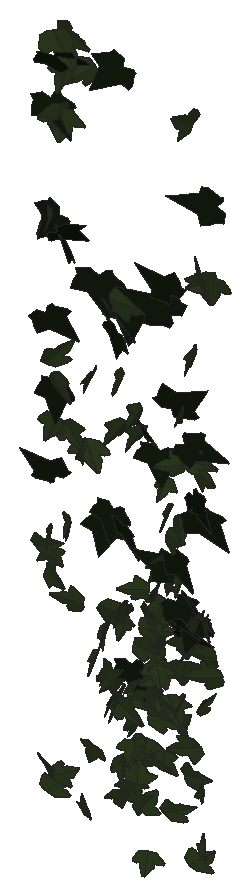
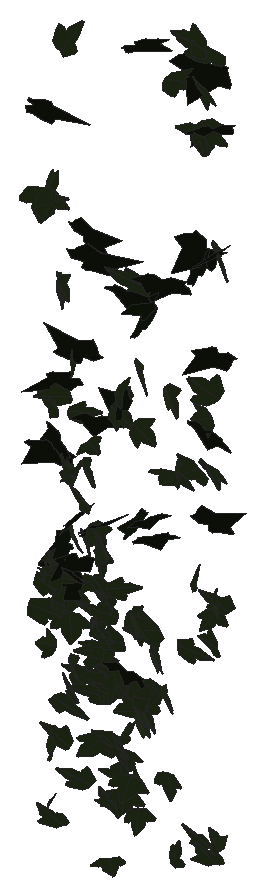
# SketchUp Ruby script. Lengths in inches.
U = 1.inch
M = Sketchup.active_model
def pt(a) = Geom::Point3d.new(a.map { |v| v * U })
def face(e, loops, mat)
  f = e.add_face(loops[0].map { |a| pt(a) })
  loops[1..].each { |l| e.add_face(l.map { |a| pt(a) }).erase! }
  f.material = f.back_material = mat if mat
  f
end
# faces: each face lists its corners as indices into pts; further lists are holes
def faces(e, pts, list, mat = nil) = list.each { |f| face(e, (f[0].is_a?(Array) ? f : [f]).map { |l| l.map { |i| pts[i] } }, mat) }
# xy, xz, yz: faces in a plane at the given z, y or x. An outline is a flat list of corners, or four numbers for a rectangle; further outlines are holes
def ring(l) = l.size == 4 ? [[l[0], l[1]], [l[2], l[1]], [l[2], l[3]], [l[0], l[3]]] : l.each_slice(2).to_a
def flat(e, list, mat, &to3) = list.each { |f| face(e, (f[0].is_a?(Array) ? f : [f]).map { |l| ring(l).map { |u, v| to3.(u, v) } }, mat) }
def xy(e, z, list, mat = nil) = flat(e, list, mat) { |x, y| [x, y, z] }
def xz(e, y, list, mat = nil) = flat(e, list, mat) { |x, z| [x, y, z] }
def yz(e, x, list, mat = nil) = flat(e, list, mat) { |y, z| [x, y, z] }
def lines(e, pts, list) = list.each { |a, b| e.add_line(pt(pts[a]), pt(pts[b])) }
# prism: a flat outline (further loops are holes) pulled along v
def prism(e, loops, v, mat = nil)
  f = face(e, loops, mat); d = Geom::Vector3d.new(v.map { |x| x * U })
  f.pushpull(f.normal.samedirection?(d) ? d.length : -d.length)
end
def box(e, o, s, mat = nil) = prism(e, [[o, [o[0] + s[0], o[1], o[2]], [o[0] + s[0], o[1] + s[1], o[2]], [o[0], o[1] + s[1], o[2]]]], [0, 0, s[2]], mat)
def at(x, y, z, deg = 0) = Geom::Transformation.translation(pt([x, y, z])) * Geom::Transformation.rotation(ORIGIN, Z_AXIS, deg.degrees)
def axes(o, x, y, z) = Geom::Transformation.new([*x, 0, *y, 0, *z, 0, *pt(o).to_a, 1])
def part(name) = M.definitions.add(name)
# library, detail: a bought-in or finely detailed component or shape, given as its bounding box
def library(name, o, s) = part(name).tap { |d| box(d.entities, o, s) }
def detail(e, o, s) = box(e.add_group.entities, o, s)
def put(e, d, t, mat = nil) = e.add_instance(d, t).tap { |i| i.material = mat if mat }
def group(e, t, mat = nil) = e.add_group.tap { |g| g.transformation = t; g.material = mat if mat }.entities
root = M.entities
M.materials.add("1026 AP 7946 SUNNY SIDE UP").color = [254, 231, 186]
M.materials.add("efeu1").color = [18, 25, 13]
M.materials.add("efeu2").color = [43, 57, 29]
c1 = part("ivyleaf_10")
p = [[0,0.5,-0.03],[-0.0625,2.02,-0.43],[-0.19,2.01,-0.46],[-0.54,1.05,-0.29],[-0.52,0.625,-0.18],[-0.83,0.76,-0.28],
  [-1.16,0.64,-0.33],[-1.15,0.33,-0.24],[-0.77,-0.39,0.02],[-0.3,-0.51,0.16],[0.04,-0.48,0.23],[-0.02,2.01,-0.4375],
  [-0.06,2.01,-0.43],[0.04,-0.49,0.23],[0.67,-0.49,0.14],[1.38,0.36,-0.2],[1.375,0.51,-0.24],[0.81,0.65,-0.19],
  [0.62,0.59,-0.15],[0.6,1.09,-0.28],[0.5,1.23,-0.31]]
faces(c1.entities,p,[[0,1,2,3,4,5,6,7,8,9,10],[11,12,0,13,14,15,16,17,18,19,20]],"efeu2")
c2 = part("ivyleaf_9")
p = [[1.54,2.16,1.25],[1.36,2.04,1.19],[-0.21,0.99,0.68],[-0.71,1.11,0.82],[-0.85,0.86,0.67],[-0.8,0.17,0.21],
  [-0.9,-0.01,0.1],[-0.67,-0.16,-0.02],[-0.08,-0.08,-0.05],[-0.03,-0.6,-0.4],[0.65,-0.88,-0.66],[0.83,-0.6,-0.49],
  [1.29,-0.42,-0.43],[1.8125,-0.07,-0.26],[1.21,0.44,0.15]]
faces(c2.entities,p,[[0,1,2,3,4,5,6,7,8,9,10,11,12,13,14]],"efeu1")
put(root,c1,axes([100.51,211.74,258.84],[-0.19659,0.09417,-0.18867],[0.19544,-0.13675,-0.16004],[-0.27947,-0.16188,0.0208]),"1026 AP 7946 SUNNY SIDE UP")
put(root,c1,axes([102.18,211.78,250.18],[0.2178,-0.07618,0.1738],[0.20785,-0.10757,-0.16206],[0.20465,0.19032,-0.02038]),"1026 AP 7946 SUNNY SIDE UP")
put(root,c1,axes([101.13,211.85,257.35],[-0.00488,-0.00097,-0.24211],[0.01134,-0.23492,-0.00047],[-0.36936,-0.0072,0.00319]),"1026 AP 7946 SUNNY SIDE UP")
put(root,c1,axes([104.76,211.65,253.64],[-0.07726,0.03119,0.21181],[-0.32666,-0.00394,-0.0506],[-0.00532,-0.21118,0.03096]),"1026 AP 7946 SUNNY SIDE UP")
put(root,c2,axes([103.46,211.8,255.27],[-0.09173,-0.23488,-0.0616],[-0.03309,-0.05498,0.24889],[-0.37914,0.06162,-0.00682]),"1026 AP 7946 SUNNY SIDE UP")
put(root,c1,axes([103.75,211.82,257.87],[-0.05406,0.02333,0.2117],[-0.12965,-0.19245,0.00718],[0.29801,-0.07949,0.04153]),"1026 AP 7946 SUNNY SIDE UP")
put(root,c1,axes([103.39,211.79,254.14],[0.1072,0.13302,-0.14483],[-0.08052,-0.13217,-0.15436],[-0.29437,0.08459,-0.01052]),"1026 AP 7946 SUNNY SIDE UP")
put(root,c1,axes([103.19,211.73,251.99],[-0.02244,0.00487,0.21035],[0.32049,-0.01245,0.01491],[0.02007,0.20428,-0.00291]),"1026 AP 7946 SUNNY SIDE UP")
put(root,c1,axes([104.73,211.79,253.09],[-0.07638,-0.01767,0.24407],[-0.28841,-0.15106,-0.05121],[0.23767,-0.18899,0.01629]),"1026 AP 7946 SUNNY SIDE UP")
put(root,c1,axes([102.57,211.88,258.71],[0.00504,-0.10131,0.23313],[0.11081,-0.2172,-0.10221],[0.37464,0.06561,0.02709]),"1026 AP 7946 SUNNY SIDE UP")
put(root,c2,axes([102.01,211.89,260.4],[-0.00288,-0.18415,0.17876],[0.01271,-0.17452,-0.1906],[0.39878,0.00423,0.00737]),"1026 AP 7946 SUNNY SIDE UP")
put(root,c1,axes([102.26,211.7,251.59],[0.18115,0.02226,0.21254],[0.32169,0.0264,-0.12055],[-0.05336,0.23471,-0.00519]),"1026 AP 7946 SUNNY SIDE UP")
put(root,c2,axes([100.59,211.91,262.14],[0.0371,-0.15314,0.23753],[0.03532,-0.23046,-0.1608],[0.43494,0.03178,-0.0072]),"1026 AP 7946 SUNNY SIDE UP")
put(root,c1,axes([101.55,211.68,250.32],[-0.2936,0.05133,0.06509],[-0.10559,-0.00902,-0.19785],[-0.07173,-0.19682,0.02481]),"1026 AP 7946 SUNNY SIDE UP")
put(root,c1,axes([102,211.79,251.66],[0.10862,-0.19941,0.06891],[0.0222,-0.06705,-0.21764],[0.33055,0.07003,-0.00803]),"1026 AP 7946 SUNNY SIDE UP")
put(root,c1,axes([103.23,211.66,254.76],[-0.00093,-0.2143,-0.09722],[-0.00318,0.09315,-0.22022],[0.36741,0.00026,-0.00215]),"1026 AP 7946 SUNNY SIDE UP")
put(root,c1,axes([103.42,211.82,254.96],[-0.03961,0.03174,0.22477],[0.27509,-0.13046,0.03963],[0.21051,0.17646,-0.00949]),"1026 AP 7946 SUNNY SIDE UP")
put(root,c1,axes([100.54,211.77,265.375],[-0.12357,-0.26188,0.04134],[0.06819,-0.05397,-0.28626],[0.44504,-0.06444,0.05534]),"1026 AP 7946 SUNNY SIDE UP")
put(root,c1,axes([100.52,211.72,267.1],[0.38789,0.09786,0.15293],[0.24346,0.0218,-0.26365],[-0.16149,0.26792,-0.03015]),"1026 AP 7946 SUNNY SIDE UP")
put(root,c1,axes([104.31,211.85,257.84],[-0.03471,-0.03254,-0.24552],[0.24332,-0.18491,0.01017],[-0.28919,-0.15168,0.03803]),"1026 AP 7946 SUNNY SIDE UP")
put(root,c2,axes([100.41,211.76,256.5],[0.04458,0.01959,0.22888],[-0.36039,0.03268,0.0252],[-0.05127,-0.21265,0.02189]),"1026 AP 7946 SUNNY SIDE UP")
put(root,c1,axes([103.47,211.82,256.69],[0.1631,-0.1985,0.09012],[0.0521,-0.08259,-0.23106],[0.33781,0.10857,-0.00787]),"1026 AP 7946 SUNNY SIDE UP")
put(root,c2,axes([102.2,211.82,255.88],[0.16159,-0.21633,0.04824],[0.01865,-0.04752,-0.24681],[0.34794,0.10301,-0.00917]),"1026 AP 7946 SUNNY SIDE UP")
put(root,c2,axes([101.79,211.86,255.75],[-0.19222,-0.20838,-0.00684],[0.01854,-0.0006,-0.24865],[0.32724,-0.12237,0.01007]),"1026 AP 7946 SUNNY SIDE UP")
put(root,c1,axes([104.52,211.65,262.59],[-0.22938,0.18916,-0.10616],[-0.07837,0.09276,0.2461],[0.33035,0.15335,-0.01533]),"1026 AP 7946 SUNNY SIDE UP")
put(root,c2,axes([100.45,211.82,258.6],[-0.28967,-0.06186,-0.17801],[0.27392,0.01655,-0.19774],[0.08918,-0.2518,0.02917]),"1026 AP 7946 SUNNY SIDE UP")
put(root,c1,axes([102.84,211.76,249.51],[-0.22155,-0.15136,0.03756],[-0.02367,-0.03686,-0.21277],[0.24398,-0.14102,0.01347]),"1026 AP 7946 SUNNY SIDE UP")
put(root,c1,axes([100.26,211.74,262.69],[0.19477,-0.23624,-0.05102],[-0.05237,0.03452,-0.28037],[0.40474,0.11815,-0.01172]),"1026 AP 7946 SUNNY SIDE UP")
put(root,c2,axes([104.03,211.73,254.78],[0.31325,-0.14847,-0.04074],[-0.06128,0.01238,-0.25553],[0.23335,0.20256,-0.01242]),"1026 AP 7946 SUNNY SIDE UP")
put(root,c2,axes([100.55,211.62,266.72],[0.38722,0.16643,-0.03986],[-0.02634,-0.04527,-0.30153],[-0.28913,0.22702,-0.02591]),"1026 AP 7946 SUNNY SIDE UP")
put(root,c1,axes([103.95,211.94,266.15],[-0.06635,-0.13772,-0.26432],[-0.13809,-0.24034,0.14682],[-0.43543,0.09721,-0.00629]),"1026 AP 7946 SUNNY SIDE UP")
put(root,c1,axes([100.11,211.71,254.69],[-0.17982,-0.02687,0.16776],[0.24101,0.06966,0.11626],[-0.12274,0.17616,-0.01749]),"1026 AP 7946 SUNNY SIDE UP")
put(root,c2,axes([103.73,211.8,253.88],[0.17427,-0.06176,0.21678],[0.24893,-0.14118,-0.1292],[0.23938,0.19177,-0.02346]),"1026 AP 7946 SUNNY SIDE UP")
put(root,c2,axes([101.91,211.875,256.11],[-0.11203,-0.23269,0.00927],[0.0058,-0.01192,-0.25067],[0.3662,-0.071,0.00681]),"1026 AP 7946 SUNNY SIDE UP")
put(root,c1,axes([100.57,211.77,265.27],[0.45415,0.06046,0.02573],[0.03947,0.00255,-0.29359],[-0.10262,0.26853,0.00093]),"1026 AP 7946 SUNNY SIDE UP")
put(root,c1,axes([100.14,211.84,249.33],[-0.17124,0.00519,0.17563],[0.23587,-0.09328,0.10112],[0.12754,0.17948,0.04881]),"1026 AP 7946 SUNNY SIDE UP")
put(root,c1,axes([104.31,211.78,254.4],[-0.00088,-0.22182,0.01479],[-0.00043,-0.01561,-0.22861],[0.34966,-0.00058,-0.00025]),"1026 AP 7946 SUNNY SIDE UP")
put(root,c1,axes([103.65,211.67,249.5],[-0.14334,-0.06132,0.18953],[0.20114,0.13428,0.11198],[-0.22987,0.15574,-0.02019]),"1026 AP 7946 SUNNY SIDE UP")
put(root,c1,axes([103.0625,211.79,250.82],[0.30307,-0.01663,-0.09637],[-0.14869,-0.01547,-0.19819],[0.01282,0.21364,-0.02059]),"1026 AP 7946 SUNNY SIDE UP")
put(root,c1,axes([103.95,211.77,253.11],[-0.30896,-0.14148,0.02035],[-0.00618,-0.02958,-0.24861],[0.22471,-0.19534,0.02114]),"1026 AP 7946 SUNNY SIDE UP")
put(root,c1,axes([100.46,211.65,259.35],[-0.0787,-0.2013,0.18006],[0.05744,0.17215,0.21465],[-0.41642,0.06179,-0.00442]),"1026 AP 7946 SUNNY SIDE UP")
put(root,c1,axes([100.375,211.8,257.78],[0.33867,-0.10946,0.00369],[-0.00857,-0.01929,-0.24301],[0.18579,0.19863,-0.01793]),"1026 AP 7946 SUNNY SIDE UP")
put(root,c1,axes([102.65,211.89,258.3],[-0.00204,-0.20535,0.15462],[0.00798,-0.15124,-0.21238],[0.40094,0.00197,0.00502]),"1026 AP 7946 SUNNY SIDE UP")
put(root,c1,axes([102.98,211.75,252.08],[-0.2792,-0.137,-0.03668],[0.06152,0.00611,-0.23019],[0.21359,-0.18084,0.01835]),"1026 AP 7946 SUNNY SIDE UP")
put(root,c1,axes([102.03,211.92,252.07],[-0.04092,-0.08914,0.21591],[-0.00538,-0.21128,-0.09402],[0.35881,-0.01333,0.02321]),"1026 AP 7946 SUNNY SIDE UP")
put(root,c1,axes([103.22,211.7,251.64],[0.01011,0.03374,0.24538],[0.33974,0.10353,-0.02053],[-0.16565,0.2144,-0.02712]),"1026 AP 7946 SUNNY SIDE UP")
put(root,c1,axes([104.08,211.87,260.64],[0.05537,-0.19387,0.11439],[0.06376,-0.10612,-0.20274],[0.34634,0.05053,0.01904]),"1026 AP 7946 SUNNY SIDE UP")
put(root,c1,axes([103.81,211.83,252.19],[0.12663,-0.19968,0.04829],[0.01411,-0.04809,-0.22188],[0.32262,0.08048,-0.00925]),"1026 AP 7946 SUNNY SIDE UP")
put(root,c1,axes([104.16,211.78,251.2],[0.18534,-0.02775,-0.19715],[-0.30132,0.01187,-0.1234],[0.03887,0.22431,-0.01653]),"1026 AP 7946 SUNNY SIDE UP")
put(root,c1,axes([103.18,211.77,252.78],[0.27617,0.09388,0.03752],[0.06025,0.00426,-0.20463],[-0.1461,0.17922,-0.01345]),"1026 AP 7946 SUNNY SIDE UP")
put(root,c1,axes([102.1,211.79,252.25],[-0.19711,-0.19958,0.0235],[-0.00224,-0.02734,-0.24258],[0.31607,-0.12466,0.01294]),"1026 AP 7946 SUNNY SIDE UP")
put(root,c1,axes([102.15,211.79,261.28],[0.02806,-0.0369,-0.28135],[0.41602,-0.07355,0.02764],[-0.1201,-0.2634,0.03]),"1026 AP 7946 SUNNY SIDE UP")
put(root,c1,axes([103.8,211.78,256.54],[0.02217,0.23158,-0.05143],[-0.00579,-0.05111,-0.23931],[-0.3729,0.01456,0.00066]),"1026 AP 7946 SUNNY SIDE UP")
put(root,c1,axes([103.94,211.77,253.69],[-0.27659,-0.11319,-0.01342],[0.03436,-0.01119,-0.21445],[0.17571,-0.17599,0.02081]),"1026 AP 7946 SUNNY SIDE UP")
put(root,c1,axes([102.71,211.72,249.98],[0.31172,0.07808,0.0062],[-0.02393,0.02354,0.21781],[0.12074,-0.19692,0.02715]),"1026 AP 7946 SUNNY SIDE UP")
put(root,c1,axes([102.87,211.85,253.88],[-0.09986,0.0072,0.24021],[0.3473,-0.07577,0.06395],[0.11783,0.22943,0.01507]),"1026 AP 7946 SUNNY SIDE UP")
put(root,c2,axes([100.6875,211.6,262.54],[0.25283,0.17394,0.10439],[0.12852,0.06073,-0.24302],[-0.28841,0.17954,-0.01678]),"1026 AP 7946 SUNNY SIDE UP")
put(root,c1,axes([102.68,211.84,250.81],[0.26439,-0.15037,0.0549],[0.04701,-0.04761,-0.23214],[0.24687,0.17011,-0.01459]),"1026 AP 7946 SUNNY SIDE UP")
put(root,c1,axes([100.62,211.83,267.24],[0.01882,-0.01234,0.27988],[0.43994,-0.03713,-0.01415],[0.06392,0.25918,0.015]),"1026 AP 7946 SUNNY SIDE UP")
put(root,c2,axes([104.7,211.84,264.4375],[-0.15463,-0.10133,-0.22898],[-0.282,-0.13182,0.14325],[-0.25958,0.20357,-0.01923]),"1026 AP 7946 SUNNY SIDE UP")
put(root,c1,axes([103.375,211.84,257.31],[0.1055,0.15917,-0.11661],[-0.07369,-0.10405,-0.17854],[-0.29899,0.08181,0.00286]),"1026 AP 7946 SUNNY SIDE UP")
put(root,c2,axes([103.65,211.78,255.6],[0.12729,-0.21417,-0.10604],[-0.06049,0.0942,-0.2353],[0.36787,0.08959,-0.002]),"1026 AP 7946 SUNNY SIDE UP")
put(root,c2,axes([102.52,211.92,258.42],[0.12413,-0.13446,0.20659],[0.1301,-0.184,-0.16111],[0.35772,0.11357,-0.01309]),"1026 AP 7946 SUNNY SIDE UP")
put(root,c2,axes([104.17,211.88,254.23],[-0.33475,-0.08786,-0.10742],[0.16729,0.01241,-0.23561],[0.13313,-0.23651,0.02597]),"1026 AP 7946 SUNNY SIDE UP")
put(root,c1,axes([102.07,211.89,251.54],[0.10893,-0.19613,0.11563],[0.04572,-0.10985,-0.21477],[0.35325,0.07469,-0.00786]),"1026 AP 7946 SUNNY SIDE UP")
put(root,c1,axes([101.31,211.76,248.63],[-0.23735,0.13346,-0.03201],[-0.02257,0.0317,0.20725],[0.21455,0.15098,-0.01361]),"1026 AP 7946 SUNNY SIDE UP")
put(root,c2,axes([102.06,211.98,266.82],[-0.28632,-0.16657,0.11656],[-0.10656,-0.0943,-0.25381],[0.29904,-0.19308,0.02116]),"1026 AP 7946 SUNNY SIDE UP")
put(root,c1,axes([100.37,211.74,248.91],[0.27742,0.02202,-0.11314],[0.16559,0.03789,0.18212],[0.06058,-0.20441,0.02032]),"1026 AP 7946 SUNNY SIDE UP")
put(root,c2,axes([100.29,211.83,265.48],[-0.03108,-0.23217,-0.13327],[0.06978,0.1177,-0.24586],[0.43928,-0.03513,0.02962]),"1026 AP 7946 SUNNY SIDE UP")
put(root,c1,axes([103.2,211.92,252.59],[0.11353,0.07899,-0.21289],[-0.19772,-0.16478,-0.11087],[-0.28702,0.14475,-0.00784]),"1026 AP 7946 SUNNY SIDE UP")
put(root,c2,axes([103.19,211.875,257.96],[-0.22069,-0.17673,-0.106],[0.11645,0.07109,-0.23172],[0.29888,-0.1582,0.01202]),"1026 AP 7946 SUNNY SIDE UP")
put(root,c1,axes([103.24,211.84,255.38],[-0.02928,-0.24532,0.03294],[-0.00141,-0.03339,-0.25364],[0.38929,-0.01857,0.00156]),"1026 AP 7946 SUNNY SIDE UP")
put(root,c1,axes([102.52,211.83,250.62],[0.33063,0.01341,-0.01591],[-0.02243,-0.01929,-0.21636],[-0.02318,0.20996,-0.01761]),"1026 AP 7946 SUNNY SIDE UP")
put(root,c1,axes([100.52,211.8,249.27],[0.19285,-0.0683,-0.1535],[0.23853,-0.02195,0.13923],[-0.09615,-0.19144,0.03752]),"1026 AP 7946 SUNNY SIDE UP")
put(root,c1,axes([103.51,211.8,252.07],[0.31385,0.08964,0.09802],[0.15167,0.01486,-0.22398],[-0.13788,0.2204,-0.02325]),"1026 AP 7946 SUNNY SIDE UP")
put(root,c1,axes([102.41,211.95,251.09],[-0.05151,0.05163,0.21344],[0.111,-0.19489,0.06048],[0.31638,0.07678,0.01353]),"1026 AP 7946 SUNNY SIDE UP")
put(root,c1,axes([100.59,211.88,266.38],[0.3722,-0.15849,0.05735],[0.05804,-0.04746,-0.28965],[0.27917,0.22117,-0.01624]),"1026 AP 7946 SUNNY SIDE UP")
put(root,c2,axes([103.43,211.85,261.4],[-0.11527,0.05112,0.29126],[-0.44654,0.02938,-0.08124],[-0.06549,-0.29031,0.0413]),"1026 AP 7946 SUNNY SIDE UP")
put(root,c2,axes([101.81,211.85,261.05],[0.2942,-0.18509,0.01369],[-0.00218,-0.02175,-0.27073],[0.2919,0.18638,-0.01582]),"1026 AP 7946 SUNNY SIDE UP")
put(root,c2,axes([101.55,211.86,261.625],[-0.21052,-0.19532,-0.16613],[0.15991,0.12423,-0.24294],[0.36354,-0.16775,0.01066]),"1026 AP 7946 SUNNY SIDE UP")
put(root,c1,axes([104.48,211.68,252.28],[0.05983,-0.11434,0.17824],[-0.03355,0.17347,0.12349],[-0.32521,-0.03893,0.02005]),"1026 AP 7946 SUNNY SIDE UP")
put(root,c2,axes([104.08,211.91,257.14],[-0.04207,-0.04472,-0.25941],[0.40154,-0.01284,-0.0257],[-0.01297,-0.25265,0.0457]),"1026 AP 7946 SUNNY SIDE UP")
put(root,c2,axes([100.27,211.73,260.35],[0.00149,-0.10637,-0.23108],[0.07652,0.21942,-0.10599],[0.38189,-0.04355,0.02214]),"1026 AP 7946 SUNNY SIDE UP")
put(root,c1,axes([102.15,211.83,259.42],[0.1703,-0.22271,-0.03426],[-0.02621,0.02747,-0.25494],[0.35281,0.10954,-0.0024]),"1026 AP 7946 SUNNY SIDE UP")
put(root,c2,axes([104.33,211.8,256.82],[-0.08339,-0.11529,-0.23252],[0.22554,0.17565,-0.1265],[0.32744,-0.15035,0.02791]),"1026 AP 7946 SUNNY SIDE UP")
put(root,c2,axes([100.31,212.04,262.6],[-0.15818,-0.19441,0.17268],[-0.07922,-0.16277,-0.22512],[0.39693,-0.10996,0.02388]),"1026 AP 7946 SUNNY SIDE UP")
put(root,c1,axes([102.18,211.88,253.55],[0.28344,-0.10037,0.05096],[0.05271,-0.04217,-0.2118],[0.16829,0.18226,-0.0195]),"1026 AP 7946 SUNNY SIDE UP")
put(root,c1,axes([104.23,211.77,248.45],[0.24739,0.00223,-0.14523],[0.21955,0.02695,0.16112],[0.03088,-0.20953,0.01793]),"1026 AP 7946 SUNNY SIDE UP")
put(root,c1,axes([101.6875,211.93,253.17],[0.12623,-0.18574,0.11864],[0.08189,-0.10405,-0.20898],[0.33464,0.09552,0.00639]),"1026 AP 7946 SUNNY SIDE UP")
put(root,c1,axes([103.4375,211.93,255.97],[0.02812,-0.07659,-0.21517],[0.2288,-0.15391,0.07023],[-0.26376,-0.14168,0.03798]),"1026 AP 7946 SUNNY SIDE UP")
put(root,c1,axes([102.16,211.93,253.85],[0.1028,-0.19996,0.11699],[0.05177,-0.1099,-0.21736],[0.35876,0.07316,-0.00216]),"1026 AP 7946 SUNNY SIDE UP")
put(root,c1,axes([101.68,211.98,252.0625],[-0.00918,0.03884,0.23108],[0.11901,-0.21105,0.03849],[0.33723,0.07554,-0.00729]),"1026 AP 7946 SUNNY SIDE UP")
put(root,c1,axes([103.19,211.79,250.63],[-0.26774,-0.09315,-0.13709],[0.20939,0.02903,-0.19708],[0.14507,-0.21382,0.03145]),"1026 AP 7946 SUNNY SIDE UP")
put(root,c1,axes([101.62,211.94,253.12],[0.16529,-0.11453,0.16348],[0.17028,-0.11689,-0.16083],[0.25732,0.15092,0.00142]),"1026 AP 7946 SUNNY SIDE UP")
put(root,c1,axes([102.67,211.88,252.16],[-0.078,0.026,0.23492],[0.35358,-0.04043,0.05494],[0.07107,0.22969,-0.01552]),"1026 AP 7946 SUNNY SIDE UP")
put(root,c1,axes([103.7,211.93,255.11],[0.20348,-0.13152,0.10932],[0.09036,-0.09244,-0.18942],[0.25068,0.14008,-0.02046]),"1026 AP 7946 SUNNY SIDE UP")
put(root,c1,axes([102.79,211.8,249.3125],[0.2992,-0.04278,-0.08904],[0.14166,0.01211,0.19877],[-0.05314,-0.20854,0.02854]),"1026 AP 7946 SUNNY SIDE UP")
put(root,c2,axes([102.33,211.93,261.12],[-0.27404,-0.13658,-0.13616],[0.20407,0.04408,-0.22428],[0.21717,-0.21377,0.03893]),"1026 AP 7946 SUNNY SIDE UP")
put(root,c1,axes([100.61,212,255.23],[-0.04886,0.00771,0.23901],[0.19483,-0.19734,0.0227],[0.30858,0.12581,0.02351]),"1026 AP 7946 SUNNY SIDE UP")
put(root,c1,axes([102.86,211.86,248.07],[0.22496,0.13868,-0.0393],[-0.03083,-0.03561,-0.20512],[-0.22438,0.14393,-0.01121]),"1026 AP 7946 SUNNY SIDE UP")
put(root,c1,axes([102.68,211.74,251.89],[0.1996,-0.01023,-0.19223],[0.26432,0.10466,0.11254],[0.12818,-0.19989,0.06727]),"1026 AP 7946 SUNNY SIDE UP")
put(root,c1,axes([102.04,211.98,258.16],[-0.04366,-0.19342,0.16214],[-0.01124,-0.15878,-0.20185],[0.39303,-0.02603,0.01224]),"1026 AP 7946 SUNNY SIDE UP")
put(root,c1,axes([104.18,211.77,260.6875],[0.07283,-0.22105,-0.13818],[-0.04184,0.13018,-0.2319],[0.40337,0.05341,0.00089]),"1026 AP 7946 SUNNY SIDE UP")
put(root,c1,axes([104.24,212.01,250.15],[0.00311,-0.00945,-0.22266],[-0.00661,-0.21605,0.00843],[-0.34002,0.00411,-0.0022]),"1026 AP 7946 SUNNY SIDE UP")
put(root,c1,axes([103.84,211.79,259.26],[0.08813,-0.22172,-0.11732],[0.00656,0.11627,-0.23299],[0.39098,0.04803,0.03036]),"1026 AP 7946 SUNNY SIDE UP")
put(root,c1,axes([102.99,211.89,254.94],[0.07859,-0.20882,-0.0471],[0.03202,-0.04087,0.22071],[-0.3342,-0.05302,0.01007]),"1026 AP 7946 SUNNY SIDE UP")
put(root,c2,axes([102.44,211.89,252.51],[-0.19599,-0.08472,-0.19613],[0.26978,0.08319,-0.15376],[0.18473,-0.21137,0.01647]),"1026 AP 7946 SUNNY SIDE UP")
put(root,c1,axes([102.12,211.91,251.81],[0.0947,-0.2001,0.04596],[0.00974,-0.04589,-0.21542],[0.32261,0.06012,-0.00699]),"1026 AP 7946 SUNNY SIDE UP")
put(root,c1,axes([103.0625,211.78,252.73],[-0.07977,-0.04383,-0.2091],[0.30375,0.06598,-0.06411],[0.1187,-0.19828,0.02354]),"1026 AP 7946 SUNNY SIDE UP")
put(root,c1,axes([103.83,211.88,256.43],[0.0692,-0.21442,-0.01693],[0.03004,-0.01157,0.2248],[-0.33666,-0.0451,0.01658]),"1026 AP 7946 SUNNY SIDE UP")
put(root,c1,axes([102.23,211.86,253.82],[-0.09521,-0.20384,-0.01599],[0.02251,0.01072,-0.21873],[0.32053,-0.0613,0.01061]),"1026 AP 7946 SUNNY SIDE UP")
put(root,c2,axes([103.73,211.79,254.54],[0.00645,-0.14884,-0.20545],[0.02002,0.19848,-0.15182],[0.38971,-0.00773,0.0112]),"1026 AP 7946 SUNNY SIDE UP")
put(root,c1,axes([104.06,211.99,253.55],[0.02509,-0.12731,0.16941],[0.01383,-0.16509,-0.13293],[0.32761,0.01672,-0.00736]),"1026 AP 7946 SUNNY SIDE UP")
put(root,c1,axes([102.15,211.85,249.38],[-0.16313,-0.1763,-0.02604],[0.03942,0.01334,-0.21011],[0.27704,-0.10571,0.01456]),"1026 AP 7946 SUNNY SIDE UP")
put(root,c1,axes([100.95,211.875,253.55],[-0.01227,0.02007,0.22315],[-0.3272,-0.0635,-0.00204],[0.09912,-0.20713,0.02091]),"1026 AP 7946 SUNNY SIDE UP")
put(root,c1,axes([104.43,212.04,262.43],[0.04057,0.00857,-0.26587],[-0.21026,-0.22149,-0.02265],[-0.34743,0.13504,-0.01734]),"1026 AP 7946 SUNNY SIDE UP")
put(root,c1,axes([102.68,211.84,253.08],[0.03869,0.02224,0.21792],[0.32428,0.04908,-0.02976],[-0.08101,0.20709,-0.01505]),"1026 AP 7946 SUNNY SIDE UP")
put(root,c1,axes([101.1875,211.95,257.39],[-0.3644,-0.08366,-0.08934],[0.19876,-0.14,-0.17641],[0.01459,-0.18239,0.17181]),"1026 AP 7946 SUNNY SIDE UP")
put(root,c1,axes([103.98,211.875,250.39],[-0.13361,0.01456,0.21069],[0.32223,0.00948,0.08711],[-0.00502,0.22119,-0.0163]),"1026 AP 7946 SUNNY SIDE UP")
put(root,c1,axes([100.1,212,254.9],[0.09203,-0.10961,0.186],[0.15819,-0.15101,-0.12848],[0.29298,0.11596,0.01094]),"1026 AP 7946 SUNNY SIDE UP")
put(root,c1,axes([104.55,211.73,254.23],[-0.09665,0.10989,0.17771],[-0.16031,0.13895,-0.12826],[-0.27786,-0.11839,0.01218]),"1026 AP 7946 SUNNY SIDE UP")
put(root,c1,axes([100.67,211.89,257.67],[0.27927,-0.00577,0.17259],[0.27393,0.00271,-0.17608],[0.00376,0.23037,0.00961]),"1026 AP 7946 SUNNY SIDE UP")
put(root,c1,axes([101.3125,211.92,259.1875],[0.06097,-0.24142,0.02657],[-0.00121,-0.02763,-0.252],[0.382,0.03845,-0.00504]),"1026 AP 7946 SUNNY SIDE UP")
put(root,c1,axes([104.08,211.78,258.1],[0.03865,0.04808,0.21083],[0.23749,0.13889,-0.05156],[-0.22933,0.15194,-0.01787]),"1026 AP 7946 SUNNY SIDE UP")
put(root,c2,axes([103.5,211.8125,261.93],[-0.04126,0.04258,0.25506],[-0.31061,0.1499,-0.0473],[-0.24344,-0.19848,0.01712]),"1026 AP 7946 SUNNY SIDE UP")
put(root,c2,axes([103.6,211.82,259.21],[-0.13358,0.04253,0.25206],[0.36927,-0.06953,0.09614],[0.1258,0.24925,-0.01458]),"1026 AP 7946 SUNNY SIDE UP")
put(root,c1,axes([100.26,211.83,254.52],[-0.18464,-0.1211,-0.09821],[0.13495,0.04852,-0.17178],[0.21788,-0.13268,0.02318]),"1026 AP 7946 SUNNY SIDE UP")
put(root,c1,axes([103.23,211.8125,253.26],[0.09553,-0.06827,-0.18976],[-0.22375,0.11705,-0.09255],[0.21213,0.1542,-0.01216]),"1026 AP 7946 SUNNY SIDE UP")
put(root,c2,axes([104.02,211.74,258.49],[0.15531,-0.06398,-0.24084],[0.03571,0.25344,-0.06019],[0.37889,0.00234,0.10439]),"1026 AP 7946 SUNNY SIDE UP")
put(root,c1,axes([104.29,211.96,254.05],[-0.00202,0.02838,0.22174],[-0.2583,-0.14061,0.01728],[0.22281,-0.16275,0.02204]),"1026 AP 7946 SUNNY SIDE UP")
put(root,c1,axes([102.66,211.84,252.2],[-0.15077,-0.19628,-0.0864],[0.08947,0.06385,-0.22356],[0.32276,-0.10938,0.02161]),"1026 AP 7946 SUNNY SIDE UP")
put(root,c1,axes([103.67,211.95,251.53],[0.17566,-0.13811,-0.13065],[0.13933,-0.09018,0.18219],[-0.25889,-0.14224,0.0094]),"1026 AP 7946 SUNNY SIDE UP")
put(root,c1,axes([103.18,211.91,254.32],[0.29989,-0.03345,-0.06564],[-0.10368,-0.01024,-0.19843],[0.04467,0.20076,-0.01984]),"1026 AP 7946 SUNNY SIDE UP")
put(root,c1,axes([102.45,211.87,249.7],[-0.26872,-0.11467,-0.03362],[0.05534,0.00479,-0.21139],[0.17882,-0.1738,0.01489]),"1026 AP 7946 SUNNY SIDE UP")
put(root,c1,axes([104.46,211.75,248.71],[-0.02426,0.14212,-0.16123],[-0.03594,0.15569,0.14812],[0.3314,0.02729,0.00426]),"1026 AP 7946 SUNNY SIDE UP")
put(root,c1,axes([101.76,211.89,253.68],[-0.16665,0.00045,-0.21702],[0.32704,-0.03722,-0.1081],[-0.05259,-0.23286,0.01547]),"1026 AP 7946 SUNNY SIDE UP")
put(root,c1,axes([102.6,212.01,254.37],[-0.01741,0.03664,0.20895],[-0.13773,-0.18447,0.02835],[0.293,-0.08454,0.02575]),"1026 AP 7946 SUNNY SIDE UP")
put(root,c1,axes([102.87,211.85,253.61],[0.0601,-0.02391,-0.23236],[0.35612,0.01349,0.03817],[0.01475,-0.22823,0.02524]),"1026 AP 7946 SUNNY SIDE UP")
put(root,c1,axes([101.35,211.99,252.36],[0.17339,-0.15358,0.11416],[0.0799,-0.10058,-0.19476],[0.28771,0.12049,-0.01472]),"1026 AP 7946 SUNNY SIDE UP")
put(root,c1,axes([101.07,212.09,266.4],[-0.1418,-0.07609,0.25972],[-0.03898,-0.26327,-0.09238],[0.4129,-0.05099,0.08047]),"1026 AP 7946 SUNNY SIDE UP")
put(root,c1,axes([100.12,211.97,253.93],[0.05566,0.00123,0.22525],[0.32539,-0.07169,-0.03452],[0.11099,0.20957,-0.01176]),"1026 AP 7946 SUNNY SIDE UP")
put(root,c1,axes([102.36,211.88,250.05],[-0.2986,-0.10444,-0.04203],[0.0695,0.00276,-0.22243],[0.16167,-0.19409,0.01799]),"1026 AP 7946 SUNNY SIDE UP")
put(root,c1,axes([103.15,212,253.27],[-0.09402,0.1386,0.17322],[0.12913,-0.14629,0.15418],[0.31634,0.10091,-0.01145]),"1026 AP 7946 SUNNY SIDE UP")
put(root,c1,axes([104.51,211.89,262.53],[-0.41641,-0.07904,0.00008],[0.01077,-0.02477,-0.28363],[0.12383,-0.26367,0.02492]),"1026 AP 7946 SUNNY SIDE UP")
